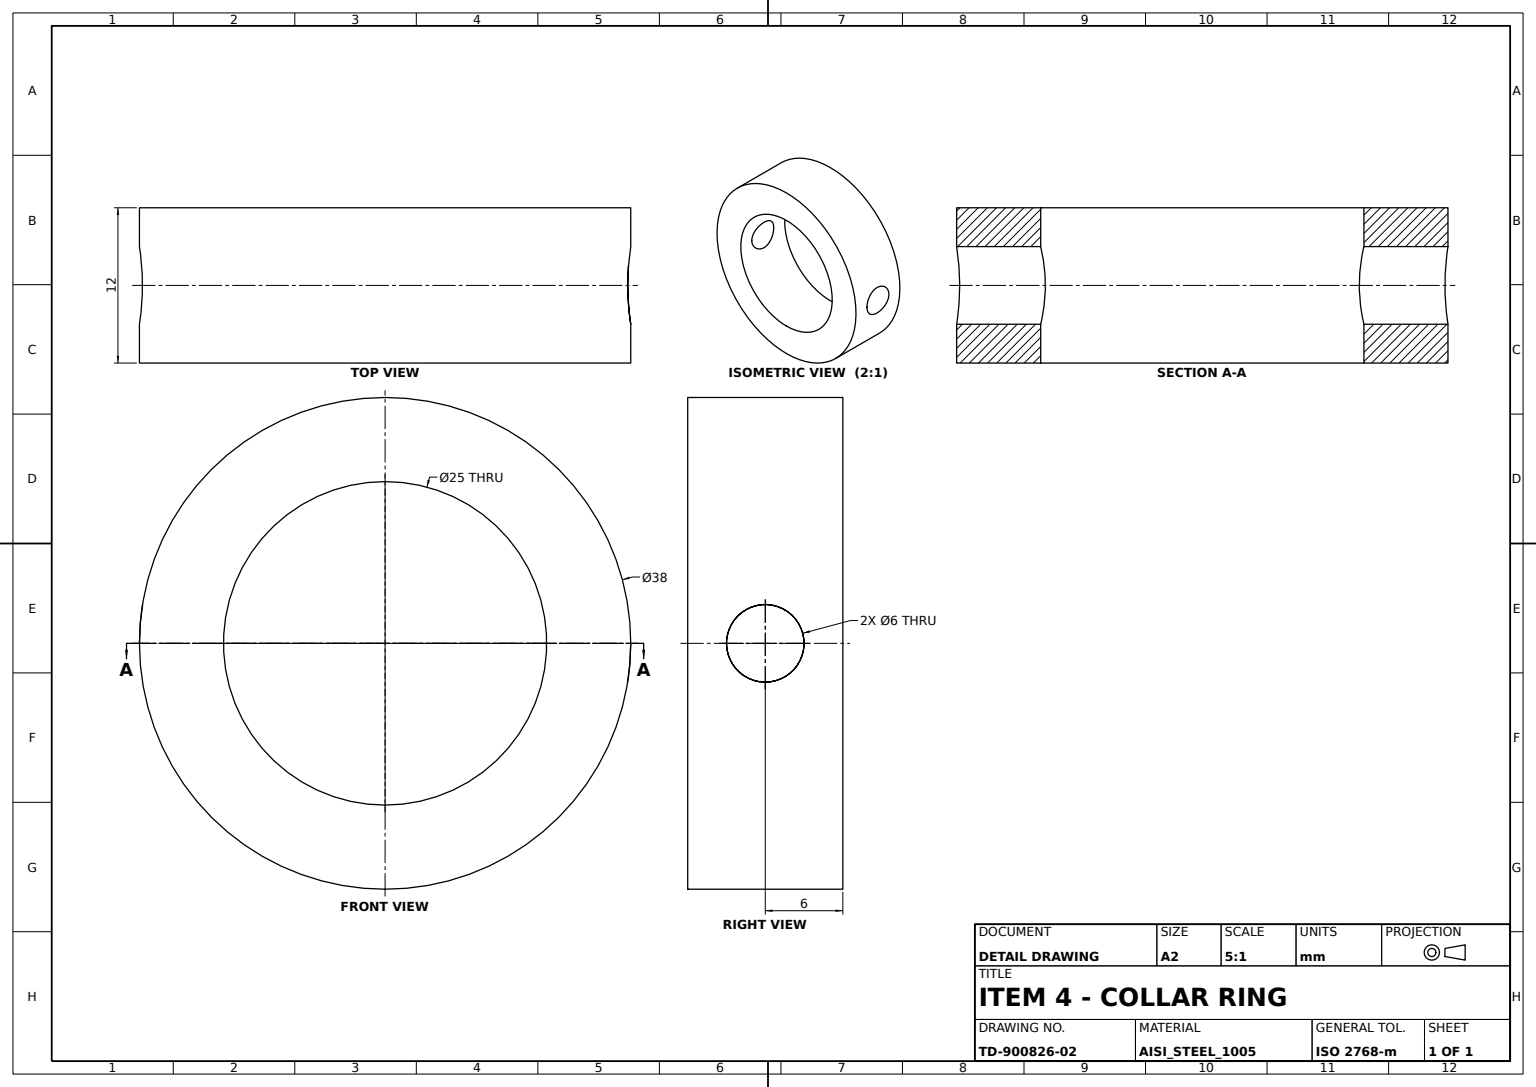
ISO-10303-21;
HEADER;
FILE_DESCRIPTION((''),'2;1');
FILE_NAME('','',(''),(''),'','','');
FILE_SCHEMA(('AUTOMOTIVE_DESIGN'));
ENDSEC;
DATA;
#1=APPLICATION_CONTEXT('');
#2=PRODUCT_CONTEXT('',#1,'mechanical');
#3=PRODUCT('','','',(#2));
#4=PRODUCT_DEFINITION_FORMATION('','',#3);
#5=PRODUCT_DEFINITION_CONTEXT('',#1,'design');
#6=PRODUCT_DEFINITION('','',#4,#5);
#7=PRODUCT_DEFINITION_SHAPE('','',#6);
#8=(LENGTH_UNIT()NAMED_UNIT(*)SI_UNIT(.MILLI.,.METRE.));
#9=(NAMED_UNIT(*)PLANE_ANGLE_UNIT()SI_UNIT($,.RADIAN.));
#10=(NAMED_UNIT(*)SI_UNIT($,.STERADIAN.)SOLID_ANGLE_UNIT());
#11=UNCERTAINTY_MEASURE_WITH_UNIT(LENGTH_MEASURE(0.005),#8,'distance_accuracy_value','');
#12=(GEOMETRIC_REPRESENTATION_CONTEXT(3)GLOBAL_UNCERTAINTY_ASSIGNED_CONTEXT((#11))GLOBAL_UNIT_ASSIGNED_CONTEXT((#8,#9,#10))REPRESENTATION_CONTEXT('',''));
#13=CARTESIAN_POINT('',(19.,0.,6.));
#14=VERTEX_POINT('',#13);
#15=CARTESIAN_POINT('',(0.,0.,6.));
#16=DIRECTION('',(0.,0.,1.));
#17=DIRECTION('',(1.,0.,0.));
#18=AXIS2_PLACEMENT_3D('',#15,#16,#17);
#19=CIRCLE('',#18,19.);
#20=EDGE_CURVE('',#14,#14,#19,.T.);
#21=ORIENTED_EDGE('',*,*,#20,.T.);
#22=EDGE_LOOP('',(#21));
#23=FACE_BOUND('',#22,.T.);
#24=CARTESIAN_POINT('',(12.5,0.,6.));
#25=VERTEX_POINT('',#24);
#26=CIRCLE('',#18,12.5);
#27=EDGE_CURVE('',#25,#25,#26,.T.);
#28=ORIENTED_EDGE('',*,*,#27,.F.);
#29=EDGE_LOOP('',(#28));
#30=FACE_BOUND('',#29,.T.);
#31=PLANE('',#18);
#32=ADVANCED_FACE('',(#23,#30),#31,.T.);
#33=CARTESIAN_POINT('',(0.,19.,3.));
#34=VERTEX_POINT('',#33);
#35=CARTESIAN_POINT('',(-2.353418,18.881288,2.348825));
#36=CARTESIAN_POINT('',(0.000563,19.059302,3.325414));
#37=CARTESIAN_POINT('',(2.351166,18.881504,2.349517));
#38=CARTESIAN_POINT('',(3.324277,18.701751,0.002857));
#39=CARTESIAN_POINT('',(2.351724,18.881472,-2.35067));
#40=CARTESIAN_POINT('',(0.000833,19.059149,-3.324014));
#41=CARTESIAN_POINT('',(-2.348081,18.881933,-2.353273));
#42=CARTESIAN_POINT('',(-3.324624,18.70169,-0.002613));
#43=B_SPLINE_CURVE_WITH_KNOTS('',3,(#35,#36,#37,#38,#39,#40,#41,#42,#35,#36,#37),.UNSPECIFIED.,.T.,.F.,(1,1,1,1,1,1,1,1,1,1,1,1,1,1,1),(-0.007044683,-0.004696455,-0.002348228,0.,0.002348228,0.004696455,0.007044683,0.00939291,0.011741138,0.014089366,0.016437593,0.018785821,0.021134048,0.023482276,0.025830503),.UNSPECIFIED.);
#44=EDGE_CURVE('',#34,#34,#43,.T.);
#45=ORIENTED_EDGE('',*,*,#44,.T.);
#46=EDGE_LOOP('',(#45));
#47=FACE_BOUND('',#46,.T.);
#48=CARTESIAN_POINT('',(0.,12.5,3.));
#49=VERTEX_POINT('',#48);
#50=CARTESIAN_POINT('',(-2.353177,12.319625,2.348756));
#51=CARTESIAN_POINT('',(0.000455,12.590122,3.325521));
#52=CARTESIAN_POINT('',(2.351355,12.319889,2.34916));
#53=CARTESIAN_POINT('',(3.324427,12.042024,0.003381));
#54=CARTESIAN_POINT('',(2.350934,12.319982,-2.35146));
#55=CARTESIAN_POINT('',(0.001353,12.589884,-3.323871));
#56=CARTESIAN_POINT('',(-2.34878,12.32048,-2.353055));
#57=CARTESIAN_POINT('',(-3.32451,12.041966,-0.001469));
#58=B_SPLINE_CURVE_WITH_KNOTS('',3,(#50,#51,#52,#53,#54,#55,#56,#57,#50,#51,#52),.UNSPECIFIED.,.T.,.F.,(1,1,1,1,1,1,1,1,1,1,1,1,1,1,1),(-0.007059428,-0.004706285,-0.002353143,0.,0.002353143,0.004706285,0.007059428,0.009412571,0.011765714,0.014118856,0.016471999,0.018825142,0.021178284,0.023531427,0.02588457),.UNSPECIFIED.);
#59=EDGE_CURVE('',#49,#49,#58,.T.);
#60=ORIENTED_EDGE('',*,*,#59,.F.);
#61=EDGE_LOOP('',(#60));
#62=FACE_BOUND('',#61,.T.);
#63=CARTESIAN_POINT('',(0.,-20.,0.));
#64=DIRECTION('',(0.,1.,0.));
#65=AXIS2_PLACEMENT_3D('',#63,#64,#16);
#66=CYLINDRICAL_SURFACE('',#65,3.);
#67=ADVANCED_FACE('',(#47,#62),#66,.F.);
#68=CARTESIAN_POINT('',(19.,0.,-6.));
#69=VERTEX_POINT('',#68);
#70=CARTESIAN_POINT('',(0.,0.,-6.));
#71=AXIS2_PLACEMENT_3D('',#70,#16,#17);
#72=CIRCLE('',#71,19.);
#73=EDGE_CURVE('',#69,#69,#72,.T.);
#74=ORIENTED_EDGE('',*,*,#73,.F.);
#75=EDGE_LOOP('',(#74));
#76=FACE_BOUND('',#75,.T.);
#77=CARTESIAN_POINT('',(12.5,0.,-6.));
#78=VERTEX_POINT('',#77);
#79=CIRCLE('',#71,12.5);
#80=EDGE_CURVE('',#78,#78,#79,.T.);
#81=ORIENTED_EDGE('',*,*,#80,.T.);
#82=EDGE_LOOP('',(#81));
#83=FACE_BOUND('',#82,.T.);
#84=PLANE('',#71);
#85=ADVANCED_FACE('',(#76,#83),#84,.F.);
#86=CARTESIAN_POINT('',(0.,-19.,3.));
#87=VERTEX_POINT('',#86);
#88=CARTESIAN_POINT('',(2.353418,-18.881288,2.348825));
#89=CARTESIAN_POINT('',(-0.000563,-19.059302,3.325414));
#90=CARTESIAN_POINT('',(-2.351166,-18.881504,2.349517));
#91=CARTESIAN_POINT('',(-3.324277,-18.701751,0.002857));
#92=CARTESIAN_POINT('',(-2.351724,-18.881472,-2.35067));
#93=CARTESIAN_POINT('',(-0.000833,-19.059149,-3.324014));
#94=CARTESIAN_POINT('',(2.348081,-18.881933,-2.353273));
#95=CARTESIAN_POINT('',(3.324624,-18.70169,-0.002613));
#96=B_SPLINE_CURVE_WITH_KNOTS('',3,(#88,#89,#90,#91,#92,#93,#94,#95,#88,#89,#90),.UNSPECIFIED.,.T.,.F.,(1,1,1,1,1,1,1,1,1,1,1,1,1,1,1),(-0.007044683,-0.004696455,-0.002348228,0.,0.002348228,0.004696455,0.007044683,0.00939291,0.011741138,0.014089366,0.016437593,0.018785821,0.021134048,0.023482276,0.025830503),.UNSPECIFIED.);
#97=EDGE_CURVE('',#87,#87,#96,.T.);
#98=ORIENTED_EDGE('',*,*,#97,.T.);
#99=EDGE_LOOP('',(#98));
#100=FACE_BOUND('',#99,.T.);
#101=CARTESIAN_POINT('',(0.,-12.5,3.));
#102=VERTEX_POINT('',#101);
#103=CARTESIAN_POINT('',(2.353177,-12.319625,2.348756));
#104=CARTESIAN_POINT('',(-0.000455,-12.590122,3.325521));
#105=CARTESIAN_POINT('',(-2.351355,-12.319889,2.34916));
#106=CARTESIAN_POINT('',(-3.324427,-12.042024,0.003381));
#107=CARTESIAN_POINT('',(-2.350934,-12.319982,-2.35146));
#108=CARTESIAN_POINT('',(-0.001353,-12.589884,-3.323871));
#109=CARTESIAN_POINT('',(2.34878,-12.32048,-2.353055));
#110=CARTESIAN_POINT('',(3.32451,-12.041966,-0.001469));
#111=B_SPLINE_CURVE_WITH_KNOTS('',3,(#103,#104,#105,#106,#107,#108,#109,#110,#103,#104,#105),.UNSPECIFIED.,.T.,.F.,(1,1,1,1,1,1,1,1,1,1,1,1,1,1,1),(-0.007059428,-0.004706285,-0.002353143,0.,0.002353143,0.004706285,0.007059428,0.009412571,0.011765714,0.014118856,0.016471999,0.018825142,0.021178284,0.023531427,0.02588457),.UNSPECIFIED.);
#112=EDGE_CURVE('',#102,#102,#111,.T.);
#113=ORIENTED_EDGE('',*,*,#112,.F.);
#114=EDGE_LOOP('',(#113));
#115=FACE_BOUND('',#114,.T.);
#116=ADVANCED_FACE('',(#100,#115),#66,.F.);
#117=ORIENTED_EDGE('',*,*,#59,.T.);
#118=EDGE_LOOP('',(#117));
#119=FACE_BOUND('',#118,.T.);
#120=ORIENTED_EDGE('',*,*,#112,.T.);
#121=EDGE_LOOP('',(#120));
#122=FACE_BOUND('',#121,.T.);
#123=ORIENTED_EDGE('',*,*,#27,.T.);
#124=EDGE_LOOP('',(#123));
#125=FACE_BOUND('',#124,.T.);
#126=ORIENTED_EDGE('',*,*,#80,.F.);
#127=EDGE_LOOP('',(#126));
#128=FACE_BOUND('',#127,.T.);
#129=DIRECTION('',(0.,0.,-1.));
#130=DIRECTION('',(-1.,0.,0.));
#131=AXIS2_PLACEMENT_3D('',#15,#129,#130);
#132=CYLINDRICAL_SURFACE('',#131,12.5);
#133=ADVANCED_FACE('',(#119,#122,#125,#128),#132,.F.);
#134=ORIENTED_EDGE('',*,*,#97,.F.);
#135=EDGE_LOOP('',(#134));
#136=FACE_BOUND('',#135,.T.);
#137=ORIENTED_EDGE('',*,*,#44,.F.);
#138=EDGE_LOOP('',(#137));
#139=FACE_BOUND('',#138,.T.);
#140=ORIENTED_EDGE('',*,*,#20,.F.);
#141=EDGE_LOOP('',(#140));
#142=FACE_BOUND('',#141,.T.);
#143=ORIENTED_EDGE('',*,*,#73,.T.);
#144=EDGE_LOOP('',(#143));
#145=FACE_BOUND('',#144,.T.);
#146=CYLINDRICAL_SURFACE('',#131,19.);
#147=ADVANCED_FACE('',(#136,#139,#142,#145),#146,.T.);
#148=CLOSED_SHELL('',(#32,#67,#85,#116,#133,#147));
#149=MANIFOLD_SOLID_BREP('',#148);
#150=ADVANCED_BREP_SHAPE_REPRESENTATION('',(#149),#12);
#151=SHAPE_DEFINITION_REPRESENTATION(#7,#150);
ENDSEC;
END-ISO-10303-21;
